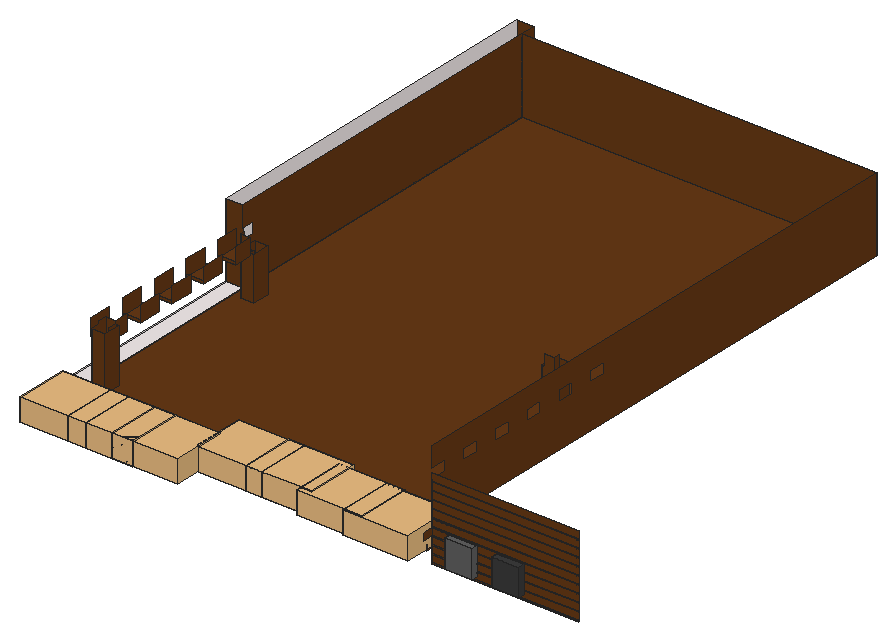
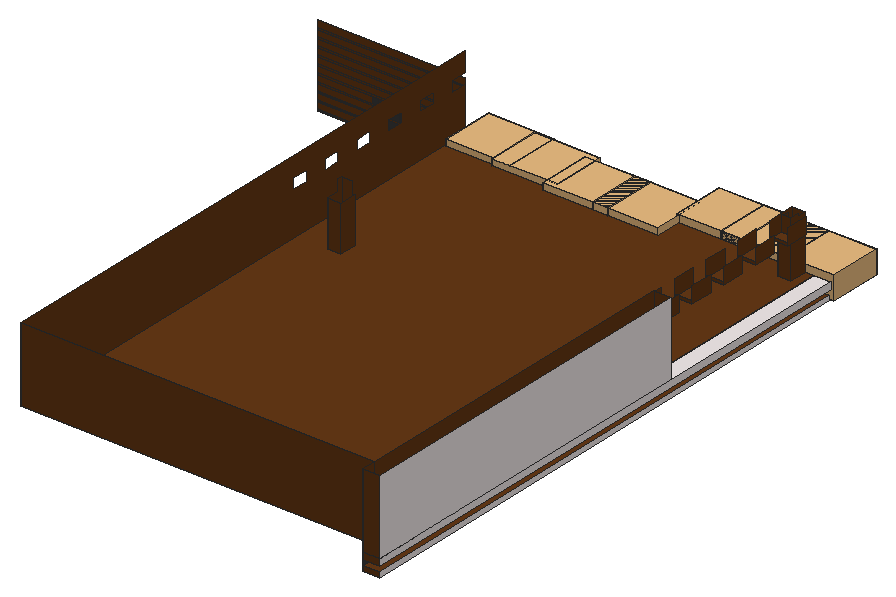
# SketchUp Ruby script. Lengths in inches.
U = 1.inch
M = Sketchup.active_model
def pt(a) = Geom::Point3d.new(a.map { |v| v * U })
def face(e, loops, mat)
  f = e.add_face(loops[0].map { |a| pt(a) })
  loops[1..].each { |l| e.add_face(l.map { |a| pt(a) }).erase! }
  f.material = f.back_material = mat if mat
  f
end
# faces: each face lists its corners as indices into pts; further lists are holes
def faces(e, pts, list, mat = nil) = list.each { |f| face(e, (f[0].is_a?(Array) ? f : [f]).map { |l| l.map { |i| pts[i] } }, mat) }
# xy, xz, yz: faces in a plane at the given z, y or x. An outline is a flat list of corners, or four numbers for a rectangle; further outlines are holes
def ring(l) = l.size == 4 ? [[l[0], l[1]], [l[2], l[1]], [l[2], l[3]], [l[0], l[3]]] : l.each_slice(2).to_a
def flat(e, list, mat, &to3) = list.each { |f| face(e, (f[0].is_a?(Array) ? f : [f]).map { |l| ring(l).map { |u, v| to3.(u, v) } }, mat) }
def xy(e, z, list, mat = nil) = flat(e, list, mat) { |x, y| [x, y, z] }
def xz(e, y, list, mat = nil) = flat(e, list, mat) { |x, z| [x, y, z] }
def yz(e, x, list, mat = nil) = flat(e, list, mat) { |y, z| [x, y, z] }
def lines(e, pts, list) = list.each { |a, b| e.add_line(pt(pts[a]), pt(pts[b])) }
# prism: a flat outline (further loops are holes) pulled along v
def prism(e, loops, v, mat = nil)
  f = face(e, loops, mat); d = Geom::Vector3d.new(v.map { |x| x * U })
  f.pushpull(f.normal.samedirection?(d) ? d.length : -d.length)
end
def box(e, o, s, mat = nil) = prism(e, [[o, [o[0] + s[0], o[1], o[2]], [o[0] + s[0], o[1] + s[1], o[2]], [o[0], o[1] + s[1], o[2]]]], [0, 0, s[2]], mat)
def at(x, y, z, deg = 0) = Geom::Transformation.translation(pt([x, y, z])) * Geom::Transformation.rotation(ORIGIN, Z_AXIS, deg.degrees)
def axes(o, x, y, z) = Geom::Transformation.new([*x, 0, *y, 0, *z, 0, *pt(o).to_a, 1])
def part(name) = M.definitions.add(name)
# library, detail: a bought-in or finely detailed component or shape, given as its bounding box
def library(name, o, s) = part(name).tap { |d| box(d.entities, o, s) }
def detail(e, o, s) = box(e.add_group.entities, o, s)
def put(e, d, t, mat = nil) = e.add_instance(d, t).tap { |i| i.material = mat if mat }
def group(e, t, mat = nil) = e.add_group.tap { |g| g.transformation = t; g.material = mat if mat }.entities
root = M.entities
M.materials.add("Generic").color = [102, 57, 22]
M.materials.add("Generic\#1").color = [96, 96, 96]
M.materials.add("Generic\#2").color = [59, 59, 59]
M.materials.add("Generic\#3").color = [243, 235, 235]
c1 = library("Plante \#58",[-0.43,-1.58,0],[20.84,18.06,17.59])
xy(root,434.875,[[288.56,54.375,403,54.68]],"Generic")
xy(root,435.875,[[288.56,54.375,403,54.68]],"Generic")
xy(root,438.4375,[[302.57,49.5625,323.88,54.375]],"Generic\#1")
xy(root,438.4375,[[339.38,49.5625,360.7,54.375]],"Generic\#2")
xy(root,441.1875,[[288.56,54.375,302.57,54.68],[323.88,54.375,339.38,54.68],[360.7,54.375,403,54.68]],"Generic")
xy(root,442.1875,[[288.56,54.375,302.57,54.68],[323.88,54.375,339.38,54.68],[360.7,54.375,403,54.68]],"Generic")
xy(root,442.58,[[200.32,54.375,201.05,62.9375],[217.69,54.375,218.42,62.9375],[248.26,54.375,248.99,62.9375],[265.63,54.375,266.36,62.9375]],"Generic")
xy(root,443.48,[[200.27,54.375,201.1,58.5625],[217.64,54.375,218.48,58.5625],[248.2,54.375,249.04,58.5625],[265.58,54.375,266.41,58.5625]],"Generic")
xy(root,446.16,[[1.33,49.51,0,498.375,13.1875,498.375,13.1875,54.375,288.56,54.375,288.56,49.625,60.27,49.625,48.53,49.51],[13.1875,54.375,288.56,58.5625]],"Generic")
xy(root,447.5,[[288.56,54.375,302.57,54.68],[323.88,54.375,339.38,54.68],[360.7,54.375,403,54.68]],"Generic")
xy(root,448.5,[[288.56,54.375,302.57,54.68],[323.88,54.375,339.38,54.68],[360.7,54.375,403,54.68]],"Generic")
xy(root,449.97,[[1.33,49.51,48.53,49.51,60.27,49.625,288.56,49.625,288.56,54.375,13.1875,54.375,13.1875,498.375,0,498.375]],"Generic")
xy(root,451.375,[[47.2,40.9375,60.27,47.4375]])
xy(root,453.8125,[[288.56,54.375,302.57,54.68],[323.88,54.375,339.38,54.68],[360.7,54.375,403,54.68]],"Generic")
xy(root,454.8125,[[288.56,54.375,302.57,54.68],[323.88,54.375,339.38,54.68],[360.7,54.375,403,54.68]],"Generic")
xy(root,459.5,[[[13.1875,54.375,288.56,486.875],[19.57,60.38,30.01,73.95],[19.57,205.01,30.01,218.57],[253.89,205.01,264.32,218.57]],[0,215.5,13.1875,498.375]],"Generic")
xy(root,459.75,[[302.57,49.5625,323.88,54.375]],"Generic\#1")
xy(root,459.75,[[339.38,49.5625,360.7,54.375]],"Generic\#2")
xy(root,460.125,[[288.56,54.375,403,54.68]],"Generic")
xy(root,461.125,[[288.56,54.375,403,54.68]],"Generic")
xy(root,466.4375,[[288.56,54.375,403,54.68]],"Generic")
xy(root,467.4375,[[288.56,54.375,403,54.68]],"Generic")
xy(root,472.75,[[288.56,54.375,403,54.68]],"Generic")
xy(root,473.75,[[288.56,54.375,403,54.68]],"Generic")
xy(root,479.0625,[[288.56,54.375,403,54.68]],"Generic")
xy(root,480.0625,[[288.56,54.375,403,54.68]],"Generic")
xy(root,485.375,[[288.56,54.375,403,54.68]],"Generic")
xy(root,486.375,[[288.56,54.375,403,54.68]],"Generic")
xy(root,491.3125,[[13.1875,67.5625,27.12,85.25],[13.1875,98.4375,27.12,116.125],[13.1875,129.3125,27.12,147],[13.1875,160.1875,27.12,177.875],[13.1875,191.0625,27.12,208.75]],"Generic")
xy(root,491.6875,[[288.56,54.375,403,54.68]],"Generic")
xy(root,492.6875,[[288.56,54.375,403,54.68]],"Generic")
xz(root,47.4375,[[47.2,451.375,60.27,454],[47.2,454,60.27,459.5]])
xz(root,49.51,[[1.33,446.16,48.53,449.97]],"Generic\#3")
xz(root,49.5625,[[302.57,438.4375,323.88,459.75]],"Generic\#1")
xz(root,49.5625,[[339.38,438.4375,360.7,459.75]],"Generic\#2")
xz(root,49.625,[[60.27,446.16,288.56,449.97]],"Generic\#3")
xz(root,54.375,[[288.56,435.875,403,435.875,403,441.1875,360.7,441.1875,360.7,438.4375,339.38,438.4375,339.38,441.1875,323.88,441.1875,323.88,438.4375,302.57,438.4375,302.57,441.1875,288.56,441.1875],[302.57,441.1875,323.88,442.1875],[339.38,441.1875,360.7,442.1875],[288.56,442.1875,302.57,447.5],[323.88,442.1875,339.38,447.5],
  [360.7,442.1875,403,447.5],[13.1875,446.16,288.56,449.97],[302.57,447.5,323.88,448.5],[339.38,447.5,360.7,448.5],[288.56,448.5,302.57,453.8125],
  [323.88,448.5,339.38,453.8125],[360.7,448.5,403,453.8125],[302.57,453.8125,323.88,454.8125],[339.38,453.8125,360.7,454.8125],[13.1875,454,288.56,459.5],
  [288.56,454.8125,302.57,454.8125,302.57,459.75,323.88,459.75,323.88,454.8125,339.38,454.8125,339.38,459.75,360.7,459.75,360.7,454.8125,403,454.8125,403,460.125,288.56,460.125],[288.56,461.125,403,466.4375],[288.56,467.4375,403,472.75],[288.56,473.75,403,479.0625],[288.56,480.0625,403,485.375],
  [288.56,486.375,403,491.6875],[288.56,492.6875,403,498]],"Generic")
xz(root,54.375,[[13.1875,449.97,288.56,454]],"Generic\#2")
xz(root,54.68,[[288.56,434.875,403,435.875],[288.56,441.1875,302.57,442.1875],[323.88,441.1875,339.38,442.1875],[360.7,441.1875,403,442.1875],[288.56,447.5,302.57,448.5],
  [323.88,447.5,339.38,448.5],[360.7,447.5,403,448.5],[288.56,453.8125,302.57,454.8125],[323.88,453.8125,339.38,454.8125],[360.7,453.8125,403,454.8125],
  [288.56,460.125,403,461.125],[288.56,466.4375,403,467.4375],[288.56,472.75,403,473.75],[288.56,479.0625,403,480.0625],[288.56,485.375,403,486.375],
  [288.56,491.6875,403,492.6875]],"Generic")
xz(root,60.38,[[19.57,459.5,30.01,501.48]],"Generic")
xz(root,67.5625,[[13.1875,491.3125,27.12,493.4375]],"Generic")
xz(root,73.95,[[19.57,459.5,19.57,503.72,27.12,503.72,27.12,501.48,30.01,501.48,30.01,459.5]],"Generic")
xz(root,85.25,[[13.1875,491.3125,27.12,493.4375]],"Generic")
xz(root,98.4375,[[13.1875,491.3125,27.12,493.4375]],"Generic")
xz(root,116.125,[[13.1875,491.3125,27.12,493.4375]],"Generic")
xz(root,129.3125,[[13.1875,491.3125,27.12,493.4375]],"Generic")
xz(root,147,[[13.1875,491.3125,27.12,493.4375]],"Generic")
xz(root,160.1875,[[13.1875,491.3125,27.12,493.4375]],"Generic")
xz(root,177.875,[[13.1875,491.3125,27.12,493.4375]],"Generic")
xz(root,191.0625,[[13.1875,491.3125,27.12,493.4375]],"Generic")
xz(root,205.01,[[19.57,459.5,30.01,459.5,30.01,493.22,27.12,493.22,27.12,503.72,19.57,503.72],[253.89,459.5,264.32,459.5,264.32,503.72,256.5625,503.72,256.5625,494.78,253.89,494.78]],"Generic")
xz(root,208.75,[[13.1875,491.3125,13.1875,493.4375,19.57,493.4375,19.57,493.22,27.12,493.22,27.12,491.3125]],"Generic")
xz(root,215.5,[[0,459.5,13.1875,517.125]],"Generic")
xz(root,218.57,[[19.57,459.5,30.01,493.22],[253.89,459.5,264.32,494.78]],"Generic")
xz(root,486.875,[[13.1875,459.5,288.56,517.125]],"Generic")
xz(root,498.375,[[0,446.16,13.1875,449.97],[0,454,13.1875,459.5],[0,459.5,13.1875,517.125]],"Generic")
yz(root,0,[[215.5,459.5,498.375,517.125]],"Generic\#3")
yz(root,13.1875,[[54.375,446.16,498.375,449.97],[54.375,454,486.875,459.5],[486.875,454,498.375,459.5],[215.5,459.5,486.875,459.5,486.875,517.125,215.5,517.125,215.5,501.6,224.75,501.6,224.75,493.4375,215.5,493.4375],[486.875,459.5,498.375,517.125],
  [67.5625,491.3125,85.25,503.72],[98.4375,491.3125,116.125,503.72],[129.3125,491.3125,147,503.72],[160.1875,491.3125,177.875,503.72],[191.0625,491.3125,208.75,503.72]],"Generic")
yz(root,13.1875,[[54.375,449.97,498.375,454]],"Generic\#2")
yz(root,19.57,[[60.38,459.5,60.38,501.48,67.5625,501.48,67.5625,503.72,73.95,503.72,73.95,459.5],[205.01,459.5,205.01,503.72,208.75,503.72,208.75,493.22,218.57,493.22,218.57,459.5]],"Generic")
yz(root,27.12,[[67.5625,491.3125,85.25,491.3125,85.25,503.72,73.95,503.72,73.95,501.48,67.5625,501.48],[98.4375,491.3125,116.125,503.72],[129.3125,491.3125,147,503.72],[160.1875,491.3125,177.875,503.72],[191.0625,491.3125,208.75,491.3125,208.75,493.22,205.01,493.22,205.01,503.72,191.0625,503.72]],"Generic")
yz(root,30.01,[[60.38,459.5,73.95,501.48],[205.01,459.5,218.57,493.22]],"Generic")
yz(root,253.89,[[205.01,459.5,218.57,494.78]],"Generic")
yz(root,264.32,[[205.01,459.5,218.57,459.5,218.57,494.78,208.75,494.78,208.75,503.72,205.01,503.72]],"Generic")
yz(root,288.56,[[54.375,434.875,54.68,435.875],[54.68,434.875,58.5625,435.875],[54.375,435.875,58.5625,441.1875],[54.375,441.1875,54.68,442.1875],[54.68,441.1875,58.5625,442.1875],
  [54.375,442.1875,58.5625,446.16],[54.375,447.5,54.68,448.5],[54.375,453.8125,54.68,454.8125],[47.4375,454,54.375,459.5],[[54.375,459.5,54.375,460.125,54.68,460.125,54.68,461.125,54.375,461.125,54.375,466.4375,54.68,466.4375,54.68,467.4375,54.375,467.4375,54.375,472.75,54.68,472.75,54.68,473.75,54.375,473.75,54.375,479.0625,54.68,479.0625,54.68,480.0625,54.375,480.0625,54.375,485.375,54.68,485.375,54.68,486.375,54.375,486.375,54.375,491.6875,54.68,491.6875,54.68,492.6875,54.375,492.6875,54.375,493.4375,67.5625,493.4375,67.5625,501.6,54.375,501.6,54.375,504.3125,54.68,504.3125,54.68,505.3125,54.375,505.3125,54.375,510.625,54.68,510.625,54.68,511.625,54.375,511.625,54.375,517.125,486.875,517.125,486.875,459.5],[208.75,493.4375,221.9375,501.6],[177.875,493.4375,191.0625,501.6],[147,493.4375,160.1875,501.6],[116.125,493.4375,129.3125,501.6],[85.25,493.4375,98.4375,501.6]]],"Generic")
yz(root,302.57,[[54.375,441.1875,54.68,442.1875],[54.375,447.5,54.68,448.5],[54.375,453.8125,54.68,454.8125]],"Generic")
yz(root,302.57,[[49.5625,438.4375,54.375,459.75]],"Generic\#1")
yz(root,323.88,[[54.375,441.1875,54.68,442.1875],[54.375,447.5,54.68,448.5],[54.375,453.8125,54.68,454.8125]],"Generic")
yz(root,323.88,[[49.5625,438.4375,54.375,459.75]],"Generic\#1")
yz(root,339.38,[[54.375,441.1875,54.68,442.1875],[54.375,447.5,54.68,448.5],[54.375,453.8125,54.68,454.8125]],"Generic")
yz(root,339.38,[[49.5625,438.4375,54.375,459.75]],"Generic\#2")
yz(root,360.7,[[54.375,441.1875,54.68,442.1875],[54.375,447.5,54.68,448.5],[54.375,453.8125,54.68,454.8125]],"Generic")
yz(root,360.7,[[49.5625,438.4375,54.375,459.75]],"Generic\#2")
yz(root,403,[[54.375,434.875,54.68,435.875],[54.375,441.1875,54.68,442.1875],[54.375,447.5,54.68,448.5],[54.375,453.8125,54.68,454.8125],[54.375,460.125,54.68,461.125],
  [54.375,466.4375,54.68,467.4375],[54.375,472.75,54.68,473.75],[54.375,479.0625,54.68,480.0625],[54.375,485.375,54.68,486.375],[54.375,491.6875,54.68,492.6875]],"Generic")
p = [[195.44,54.375,432.86],[195.87,54.375,432.27],[195.87,62.9375,432.27],[195.44,62.9375,432.86],[205.5,54.375,432.27],[205.93,54.375,432.86],
  [205.93,62.9375,432.86],[205.5,62.9375,432.27],[212.81,54.375,432.86],[213.25,54.375,432.27],[213.25,62.9375,432.27],[212.81,62.9375,432.86],
  [222.87,54.375,432.27],[223.31,54.375,432.86],[223.31,62.9375,432.86],[222.87,62.9375,432.27],[243.37,54.375,432.86],[243.81,54.375,432.27],
  [243.81,62.9375,432.27],[243.37,62.9375,432.86],[253.43,54.375,432.27],[253.87,54.375,432.86],[253.87,62.9375,432.86],[253.43,62.9375,432.27],
  [260.75,54.375,432.86],[261.18,54.375,432.27],[261.18,62.9375,432.27],[260.75,62.9375,432.86],[270.81,54.375,432.27],[271.25,54.375,432.86],
  [271.25,62.9375,432.86],[270.81,62.9375,432.27],[194.26,54.375,433.08],[194.68,54.375,432.36],[194.68,58.5625,432.36],[194.26,58.5625,433.08],
  [206.6875,54.375,432.36],[207.11,54.375,433.08],[207.11,58.5625,433.08],[206.6875,58.5625,432.36],[211.64,54.375,433.08],[212.05,54.375,432.36],
  [212.05,58.5625,432.36],[211.64,58.5625,433.08],[224.0625,54.375,432.36],[224.48,54.375,433.08],[224.48,58.5625,433.08],[224.0625,58.5625,432.36],
  [242.2,54.375,433.08],[242.62,54.375,432.36],[242.62,58.5625,432.36],[242.2,58.5625,433.08],[254.625,54.375,432.36],[255.04,54.375,433.08],
  [255.04,58.5625,433.08],[254.625,58.5625,432.36],[259.57,54.375,433.08],[259.99,54.375,432.36],[259.99,58.5625,432.36],[259.57,58.5625,433.08],
  [272,54.375,432.36],[272.42,54.375,433.08],[272.42,58.5625,433.08],[272,58.5625,432.36],[195.07,54.375,433.49],[195.07,62.9375,433.49],
  [206.3,54.375,433.49],[206.3,62.9375,433.49],[212.44,54.375,433.49],[212.44,62.9375,433.49],[223.67,54.375,433.49],[223.67,62.9375,433.49],
  [243.01,54.375,433.49],[243.01,62.9375,433.49],[254.24,54.375,433.49],[254.24,62.9375,433.49],[260.38,54.375,433.49],[260.38,62.9375,433.49],
  [271.61,54.375,433.49],[271.61,62.9375,433.49],[193.93,54.375,433.85],[193.93,58.5625,433.85],[207.4375,54.375,433.85],[207.4375,58.5625,433.85],
  [211.31,54.375,433.85],[211.31,58.5625,433.85],[224.8125,54.375,433.85],[224.8125,58.5625,433.85],[241.87,54.375,433.85],[241.87,58.5625,433.85],
  [255.375,54.375,433.85],[255.375,58.5625,433.85],[259.24,54.375,433.85],[259.24,58.5625,433.85],[272.75,54.375,433.85],[272.75,58.5625,433.85],
  [194.78,54.375,434.16],[194.78,62.9375,434.16],[206.59,54.375,434.16],[206.59,62.9375,434.16],[212.16,54.375,434.16],[212.16,62.9375,434.16],
  [223.96,54.375,434.16],[223.96,62.9375,434.16],[242.72,54.375,434.16],[242.72,62.9375,434.16],[254.53,54.375,434.16],[254.53,62.9375,434.16],
  [260.09,54.375,434.16],[260.09,62.9375,434.16],[271.9,54.375,434.16],[271.9,62.9375,434.16],[193.69,54.375,434.65],[193.69,58.5625,434.65],
  [207.68,54.375,434.65],[207.68,58.5625,434.65],[211.07,54.375,434.65],[211.07,58.5625,434.65],[225.05,54.375,434.65],[225.05,58.5625,434.65],
  [241.63,54.375,434.65],[241.63,58.5625,434.65],[255.62,54.375,434.65],[255.62,58.5625,434.65],[259,54.375,434.65],[259,58.5625,434.65],
  [272.99,54.375,434.65],[272.99,58.5625,434.65],[194.57,54.375,434.86],[194.57,62.9375,434.86],[206.8,54.375,434.86],[206.8,62.9375,434.86],
  [211.95,54.375,434.86],[211.95,62.9375,434.86],[224.17,54.375,434.86],[224.17,62.9375,434.86],[242.51,54.375,434.86],[242.51,62.9375,434.86],
  [254.73,54.375,434.86],[254.73,62.9375,434.86],[259.88,54.375,434.86],[259.88,62.9375,434.86],[272.11,54.375,434.86],[272.11,62.9375,434.86],
  [193.55,54.375,435.47],[193.55,58.5625,435.47],[207.82,54.375,435.47],[207.82,58.5625,435.47],[210.92,54.375,435.47],[210.92,58.5625,435.47],
  [225.2,54.375,435.47],[225.2,58.5625,435.47],[241.48,54.375,435.47],[241.48,58.5625,435.47],[255.76,54.375,435.47],[255.76,58.5625,435.47],
  [258.86,54.375,435.47],[258.86,58.5625,435.47],[273.14,54.375,435.47],[273.14,58.5625,435.47],[194.44,54.375,435.58],[194.44,62.9375,435.58],
  [206.92,54.375,435.58],[206.92,62.9375,435.58],[211.82,54.375,435.58],[211.82,62.9375,435.58],[224.3,54.375,435.58],[224.3,62.9375,435.58],
  [242.38,54.375,435.58],[242.38,62.9375,435.58],[254.86,54.375,435.58],[254.86,62.9375,435.58],[259.76,54.375,435.58],[259.76,62.9375,435.58],
  [272.24,54.375,435.58],[272.24,62.9375,435.58],[193.5,54.375,436.31],[193.5,58.5625,436.31],[207.87,54.375,436.31],[207.87,58.5625,436.31],
  [210.87,54.375,436.31],[210.87,58.5625,436.31],[225.25,54.375,436.31],[225.25,58.5625,436.31],[241.43,54.375,436.31],[241.43,58.5625,436.31],
  [255.81,54.375,436.31],[255.81,58.5625,436.31],[258.81,54.375,436.31],[258.81,58.5625,436.31],[273.18,54.375,436.31],[273.18,58.5625,436.31],
  [194.4,54.375,436.31],[194.4,62.9375,436.31],[206.97,54.375,436.31],[206.97,62.9375,436.31],[211.78,54.375,436.31],[211.78,62.9375,436.31],
  [224.34,54.375,436.31],[224.34,62.9375,436.31],[242.34,54.375,436.31],[242.34,62.9375,436.31],[254.9,54.375,436.31],[254.9,62.9375,436.31],
  [259.71,54.375,436.31],[259.71,62.9375,436.31],[272.28,54.375,436.31],[272.28,62.9375,436.31],[193.55,54.375,437.14],[193.55,58.5625,437.14],
  [194.44,54.375,437.04],[194.44,62.9375,437.04],[206.92,54.375,437.04],[206.92,62.9375,437.04],[207.82,54.375,437.14],[207.82,58.5625,437.14],
  [210.92,54.375,437.14],[210.92,58.5625,437.14],[211.82,54.375,437.04],[211.82,62.9375,437.04],[224.3,54.375,437.04],[224.3,62.9375,437.04],
  [225.2,54.375,437.14],[225.2,58.5625,437.14],[241.48,54.375,437.14],[241.48,58.5625,437.14],[242.38,54.375,437.04],[242.38,62.9375,437.04],
  [254.86,54.375,437.04],[254.86,62.9375,437.04],[255.76,54.375,437.14],[255.76,58.5625,437.14],[258.86,54.375,437.14],[258.86,58.5625,437.14],
  [259.76,54.375,437.04],[259.76,62.9375,437.04],[272.24,54.375,437.04],[272.24,62.9375,437.04],[273.14,54.375,437.14],[273.14,58.5625,437.14],
  [194.57,54.375,437.76],[194.57,62.9375,437.76],[206.8,54.375,437.76],[206.8,62.9375,437.76],[211.95,54.375,437.76],[211.95,62.9375,437.76],
  [224.17,54.375,437.76],[224.17,62.9375,437.76],[242.51,54.375,437.76],[242.51,62.9375,437.76],[254.73,54.375,437.76],[254.73,62.9375,437.76],
  [259.88,54.375,437.76],[259.88,62.9375,437.76],[272.11,54.375,437.76],[272.11,62.9375,437.76],[193.69,54.375,437.97],[193.69,58.5625,437.97],
  [207.68,54.375,437.97],[207.68,58.5625,437.97],[211.07,54.375,437.97],[211.07,58.5625,437.97],[225.05,54.375,437.97],[225.05,58.5625,437.97],
  [241.63,54.375,437.97],[241.63,58.5625,437.97],[255.62,54.375,437.97],[255.62,58.5625,437.97],[259,54.375,437.97],[259,58.5625,437.97],
  [272.99,54.375,437.97],[272.99,58.5625,437.97],[194.78,54.375,438.46],[194.78,62.9375,438.46],[206.59,54.375,438.46],[206.59,62.9375,438.46],
  [212.16,54.375,438.46],[212.16,62.9375,438.46],[223.96,54.375,438.46],[223.96,62.9375,438.46],[242.72,54.375,438.46],[242.72,62.9375,438.46],
  [254.53,54.375,438.46],[254.53,62.9375,438.46],[260.09,54.375,438.46],[260.09,62.9375,438.46],[271.9,54.375,438.46],[271.9,62.9375,438.46],
  [193.93,54.375,438.77],[193.93,58.5625,438.77],[207.4375,54.375,438.77],[207.4375,58.5625,438.77],[211.31,54.375,438.77],[211.31,58.5625,438.77],
  [224.8125,54.375,438.77],[224.8125,58.5625,438.77],[241.87,54.375,438.77],[241.87,58.5625,438.77],[255.375,54.375,438.77],[255.375,58.5625,438.77],
  [259.24,54.375,438.77],[259.24,58.5625,438.77],[272.75,54.375,438.77],[272.75,58.5625,438.77],[195.07,54.375,439.13],[195.07,62.9375,439.13],
  [206.3,54.375,439.13],[206.3,62.9375,439.13],[212.44,54.375,439.13],[212.44,62.9375,439.13],[223.67,54.375,439.13],[223.67,62.9375,439.13],
  [243.01,54.375,439.13],[243.01,62.9375,439.13],[254.24,54.375,439.13],[254.24,62.9375,439.13],[260.38,54.375,439.13],[260.38,62.9375,439.13],
  [271.61,54.375,439.13],[271.61,62.9375,439.13],[194.26,54.375,439.53],[194.26,58.5625,439.53],[207.11,54.375,439.53],[207.11,58.5625,439.53],
  [211.64,54.375,439.53],[211.64,58.5625,439.53],[224.48,54.375,439.53],[224.48,58.5625,439.53],[242.2,54.375,439.53],[242.2,58.5625,439.53],
  [255.04,54.375,439.53],[255.04,58.5625,439.53],[259.57,54.375,439.53],[259.57,58.5625,439.53],[272.42,54.375,439.53],[272.42,58.5625,439.53],
  [195.44,54.375,439.76],[195.44,62.9375,439.76],[205.93,54.375,439.76],[205.93,62.9375,439.76],[212.81,54.375,439.76],[212.81,62.9375,439.76],
  [223.31,54.375,439.76],[223.31,62.9375,439.76],[243.37,54.375,439.76],[243.37,62.9375,439.76],[253.87,54.375,439.76],[253.87,62.9375,439.76],
  [260.75,54.375,439.76],[260.75,62.9375,439.76],[271.25,54.375,439.76],[271.25,62.9375,439.76],[194.68,54.375,440.26],[194.68,58.5625,440.26],
  [206.6875,54.375,440.26],[206.6875,58.5625,440.26],[212.05,54.375,440.26],[212.05,58.5625,440.26],[224.0625,54.375,440.26],[224.0625,58.5625,440.26],
  [242.62,54.375,440.26],[242.62,58.5625,440.26],[254.625,54.375,440.26],[254.625,58.5625,440.26],[259.99,54.375,440.26],[259.99,58.5625,440.26],
  [272,54.375,440.26],[272,58.5625,440.26],[195.87,54.375,440.35],[195.87,62.9375,440.35],[205.5,54.375,440.35],[205.5,62.9375,440.35],
  [213.25,54.375,440.35],[213.25,62.9375,440.35],[222.87,54.375,440.35],[222.87,62.9375,440.35],[243.81,54.375,440.35],[243.81,62.9375,440.35],
  [253.43,54.375,440.35],[253.43,62.9375,440.35],[261.18,54.375,440.35],[261.18,62.9375,440.35],[270.81,54.375,440.35],[270.81,62.9375,440.35],
  [195.18,54.375,440.93],[195.18,58.5625,440.93],[196.37,54.375,440.88],[196.37,62.9375,440.88],[205,54.375,440.88],[205,62.9375,440.88],
  [206.19,54.375,440.93],[206.19,58.5625,440.93],[212.55,54.375,440.93],[212.55,58.5625,440.93],[213.75,54.375,440.88],[213.75,62.9375,440.88],
  [222.37,54.375,440.88],[222.37,62.9375,440.88],[223.57,54.375,440.93],[223.57,58.5625,440.93],[243.12,54.375,440.93],[243.12,58.5625,440.93],
  [244.31,54.375,440.88],[244.31,62.9375,440.88],[252.93,54.375,440.88],[252.93,62.9375,440.88],[254.13,54.375,440.93],[254.13,58.5625,440.93],
  [260.49,54.375,440.93],[260.49,58.5625,440.93],[261.69,54.375,440.88],[261.69,62.9375,440.88],[270.31,54.375,440.88],[270.31,62.9375,440.88],
  [271.5,54.375,440.93],[271.5,58.5625,440.93],[195.75,54.375,441.54],[195.75,58.5625,441.54],[196.93,54.375,441.35],[196.93,62.9375,441.35],
  [204.4375,54.375,441.35],[204.4375,62.9375,441.35],[205.62,54.375,441.54],[205.62,58.5625,441.54],[213.125,54.375,441.54],[213.125,58.5625,441.54],
  [214.31,54.375,441.35],[214.31,62.9375,441.35],[221.8125,54.375,441.35],[221.8125,62.9375,441.35],[222.99,54.375,441.54],[222.99,58.5625,441.54],
  [243.6875,54.375,441.54],[243.6875,58.5625,441.54],[244.87,54.375,441.35],[244.87,62.9375,441.35],[252.375,54.375,441.35],[252.375,62.9375,441.35],
  [253.55,54.375,441.54],[253.55,58.5625,441.54],[261.0625,54.375,441.54],[261.0625,58.5625,441.54],[262.25,54.375,441.35],[262.25,62.9375,441.35],
  [269.75,54.375,441.35],[269.75,62.9375,441.35],[270.93,54.375,441.54],[270.93,58.5625,441.54],[197.54,54.375,441.75],[197.54,62.9375,441.75],
  [203.83,54.375,441.75],[203.83,62.9375,441.75],[214.92,54.375,441.75],[214.92,62.9375,441.75],[221.2,54.375,441.75],[221.2,62.9375,441.75],
  [245.48,54.375,441.75],[245.48,62.9375,441.75],[251.76,54.375,441.75],[251.76,62.9375,441.75],[262.86,54.375,441.75],[262.86,62.9375,441.75],
  [269.14,54.375,441.75],[269.14,62.9375,441.75],[196.39,54.375,442.07],[196.39,58.5625,442.07],[204.98,54.375,442.07],[204.98,58.5625,442.07],
  [213.77,54.375,442.07],[213.77,58.5625,442.07],[222.35,54.375,442.07],[222.35,58.5625,442.07],[244.33,54.375,442.07],[244.33,58.5625,442.07],
  [252.91,54.375,442.07],[252.91,58.5625,442.07],[261.7,54.375,442.07],[261.7,58.5625,442.07],[270.29,54.375,442.07],[270.29,58.5625,442.07],
  [198.2,54.375,442.08],[198.2,62.9375,442.08],[203.17,54.375,442.08],[203.17,62.9375,442.08],[215.57,54.375,442.08],[215.57,62.9375,442.08],
  [220.55,54.375,442.08],[220.55,62.9375,442.08],[246.13,54.375,442.08],[246.13,62.9375,442.08],[251.11,54.375,442.08],[251.11,62.9375,442.08],
  [263.51,54.375,442.08],[263.51,62.9375,442.08],[268.48,54.375,442.08],[268.48,62.9375,442.08],[197.09,54.375,442.53],[197.09,58.5625,442.53],
  [198.88,54.375,442.33],[198.88,62.9375,442.33],[202.49,54.375,442.33],[202.49,62.9375,442.33],[204.28,54.375,442.53],[204.28,58.5625,442.53],
  [214.47,54.375,442.53],[214.47,58.5625,442.53],[216.26,54.375,442.33],[216.26,62.9375,442.33],[219.86,54.375,442.33],[219.86,62.9375,442.33],
  [221.65,54.375,442.53],[221.65,58.5625,442.53],[245.03,54.375,442.53],[245.03,58.5625,442.53],[246.82,54.375,442.33],[246.82,62.9375,442.33],
  [250.42,54.375,442.33],[250.42,62.9375,442.33],[252.22,54.375,442.53],[252.22,58.5625,442.53],[262.4,54.375,442.53],[262.4,58.5625,442.53],
  [264.19,54.375,442.33],[264.19,62.9375,442.33],[267.8,54.375,442.33],[267.8,62.9375,442.33],[269.59,54.375,442.53],[269.59,58.5625,442.53],
  [199.59,54.375,442.5],[199.59,62.9375,442.5],[201.78,54.375,442.5],[201.78,62.9375,442.5],[216.97,54.375,442.5],[216.97,62.9375,442.5],
  [219.15,54.375,442.5],[219.15,62.9375,442.5],[247.53,54.375,442.5],[247.53,62.9375,442.5],[249.71,54.375,442.5],[249.71,62.9375,442.5],
  [264.91,54.375,442.5],[264.91,62.9375,442.5],[267.09,54.375,442.5],[267.09,62.9375,442.5],[197.84,54.375,442.91],[197.84,58.5625,442.91],
  [200.32,54.375,442.58],[200.32,62.9375,442.58],[201.05,54.375,442.58],[201.05,62.9375,442.58],[203.53,54.375,442.91],[203.53,58.5625,442.91],
  [215.21,54.375,442.91],[215.21,58.5625,442.91],[217.69,54.375,442.58],[217.69,62.9375,442.58],[218.42,54.375,442.58],[218.42,62.9375,442.58],
  [220.91,54.375,442.91],[220.91,58.5625,442.91],[245.77,54.375,442.91],[245.77,58.5625,442.91],[248.26,54.375,442.58],[248.26,62.9375,442.58],
  [248.99,54.375,442.58],[248.99,62.9375,442.58],[251.47,54.375,442.91],[251.47,58.5625,442.91],[263.15,54.375,442.91],[263.15,58.5625,442.91],
  [265.63,54.375,442.58],[265.63,62.9375,442.58],[266.36,54.375,442.58],[266.36,62.9375,442.58],[268.84,54.375,442.91],[268.84,58.5625,442.91],
  [198.62,54.375,443.19],[198.62,58.5625,443.19],[202.75,54.375,443.19],[202.75,58.5625,443.19],[216,54.375,443.19],[216,58.5625,443.19],
  [220.12,54.375,443.19],[220.12,58.5625,443.19],[246.56,54.375,443.19],[246.56,58.5625,443.19],[250.68,54.375,443.19],[250.68,58.5625,443.19],
  [263.94,54.375,443.19],[263.94,58.5625,443.19],[268.06,54.375,443.19],[268.06,58.5625,443.19],[199.4375,54.375,443.39],[199.4375,58.5625,443.39],
  [201.93,54.375,443.39],[201.93,58.5625,443.39],[216.8125,54.375,443.39],[216.8125,58.5625,443.39],[219.31,54.375,443.39],[219.31,58.5625,443.39],
  [247.375,54.375,443.39],[247.375,58.5625,443.39],[249.87,54.375,443.39],[249.87,58.5625,443.39],[264.75,54.375,443.39],[264.75,58.5625,443.39],
  [267.24,54.375,443.39],[267.24,58.5625,443.39],[200.27,54.375,443.48],[200.27,58.5625,443.48],[201.1,54.375,443.48],[201.1,58.5625,443.48],
  [217.64,54.375,443.48],[217.64,58.5625,443.48],[218.48,54.375,443.48],[218.48,58.5625,443.48],[248.2,54.375,443.48],[248.2,58.5625,443.48],
  [249.04,54.375,443.48],[249.04,58.5625,443.48],[265.58,54.375,443.48],[265.58,58.5625,443.48],[266.41,54.375,443.48],[266.41,58.5625,443.48],
  [0,498.375,449.97],[0,498.375,446.16],[1.33,49.51,446.16],[1.33,49.51,449.97],[48.53,49.51,446.16],[60.27,49.625,446.16],
  [60.27,49.625,449.97],[48.53,49.51,449.97]]
faces(root,p,[[0,1,2,3],[4,5,6,7],[8,9,10,11],[12,13,14,15],[16,17,18,19],[20,21,22,23],[24,25,26,27],[28,29,30,31],
  [32,33,34,35],[36,37,38,39],[40,41,42,43],[44,45,46,47],[48,49,50,51],[52,53,54,55],[56,57,58,59],[60,61,62,63],
  [64,0,3,65],[5,66,67,6],[68,8,11,69],[13,70,71,14],[72,16,19,73],[21,74,75,22],[76,24,27,77],[29,78,79,30],
  [80,32,35,81],[37,82,83,38],[84,40,43,85],[45,86,87,46],[88,48,51,89],[53,90,91,54],[92,56,59,93],[61,94,95,62],
  [96,64,65,97],[66,98,99,67],[100,68,69,101],[70,102,103,71],[104,72,73,105],[74,106,107,75],[108,76,77,109],[78,110,111,79],
  [112,80,81,113],[82,114,115,83],[116,84,85,117],[86,118,119,87],[120,88,89,121],[90,122,123,91],[124,92,93,125],[94,126,127,95],
  [128,96,97,129],[98,130,131,99],[132,100,101,133],[102,134,135,103],[136,104,105,137],[106,138,139,107],[140,108,109,141],[110,142,143,111],
  [144,112,113,145],[114,146,147,115],[148,116,117,149],[118,150,151,119],[152,120,121,153],[122,154,155,123],[156,124,125,157],[126,158,159,127],
  [160,128,129,161],[130,162,163,131],[164,132,133,165],[134,166,167,135],[168,136,137,169],[138,170,171,139],[172,140,141,173],[142,174,175,143],
  [176,144,145,177],[146,178,179,147],[180,148,149,181],[150,182,183,151],[184,152,153,185],[154,186,187,155],[188,156,157,189],[158,190,191,159],
  [192,160,161,193],[162,194,195,163],[196,164,165,197],[166,198,199,167],[200,168,169,201],[170,202,203,171],[204,172,173,205],[174,206,207,175],
  [208,176,177,209],[210,192,193,211],[194,212,213,195],[178,214,215,179],[216,180,181,217],[218,196,197,219],[198,220,221,199],[182,222,223,183],
  [224,184,185,225],[226,200,201,227],[202,228,229,203],[186,230,231,187],[232,188,189,233],[234,204,205,235],[206,236,237,207],[190,238,239,191],
  [240,210,211,241],[212,242,243,213],[244,218,219,245],[220,246,247,221],[248,226,227,249],[228,250,251,229],[252,234,235,253],[236,254,255,237],
  [256,208,209,257],[214,258,259,215],[260,216,217,261],[222,262,263,223],[264,224,225,265],[230,266,267,231],[268,232,233,269],[238,270,271,239],
  [272,240,241,273],[242,274,275,243],[276,244,245,277],[246,278,279,247],[280,248,249,281],[250,282,283,251],[284,252,253,285],[254,286,287,255],
  [288,256,257,289],[258,290,291,259],[292,260,261,293],[262,294,295,263],[296,264,265,297],[266,298,299,267],[300,268,269,301],[270,302,303,271],
  [304,272,273,305],[274,306,307,275],[308,276,277,309],[278,310,311,279],[312,280,281,313],[282,314,315,283],[316,284,285,317],[286,318,319,287],
  [320,288,289,321],[290,322,323,291],[324,292,293,325],[294,326,327,295],[328,296,297,329],[298,330,331,299],[332,300,301,333],[302,334,335,303],
  [336,304,305,337],[306,338,339,307],[340,308,309,341],[310,342,343,311],[344,312,313,345],[314,346,347,315],[348,316,317,349],[318,350,351,319],
  [352,320,321,353],[322,354,355,323],[356,324,325,357],[326,358,359,327],[360,328,329,361],[330,362,363,331],[364,332,333,365],[334,366,367,335],
  [368,336,337,369],[338,370,371,339],[372,340,341,373],[342,374,375,343],[376,344,345,377],[346,378,379,347],[380,348,349,381],[350,382,383,351],
  [384,352,353,385],[386,368,369,387],[370,388,389,371],[354,390,391,355],[392,356,357,393],[394,372,373,395],[374,396,397,375],[358,398,399,359],
  [400,360,361,401],[402,376,377,403],[378,404,405,379],[362,406,407,363],[408,364,365,409],[410,380,381,411],[382,412,413,383],[366,414,415,367],
  [416,384,385,417],[418,386,387,419],[388,420,421,389],[390,422,423,391],[424,392,393,425],[426,394,395,427],[396,428,429,397],[398,430,431,399],
  [432,400,401,433],[434,402,403,435],[404,436,437,405],[406,438,439,407],[440,408,409,441],[442,410,411,443],[412,444,445,413],[414,446,447,415],
  [448,418,419,449],[420,450,451,421],[452,426,427,453],[428,454,455,429],[456,434,435,457],[436,458,459,437],[460,442,443,461],[444,462,463,445],
  [464,416,417,465],[422,466,467,423],[468,424,425,469],[430,470,471,431],[472,432,433,473],[438,474,475,439],[476,440,441,477],[446,478,479,447],
  [480,448,449,481],[450,482,483,451],[484,452,453,485],[454,486,487,455],[488,456,457,489],[458,490,491,459],[492,460,461,493],[462,494,495,463],
  [496,464,465,497],[498,480,481,499],[482,500,501,483],[466,502,503,467],[504,468,469,505],[506,484,485,507],[486,508,509,487],[470,510,511,471],
  [512,472,473,513],[514,488,489,515],[490,516,517,491],[474,518,519,475],[520,476,477,521],[522,492,493,523],[494,524,525,495],[478,526,527,479],
  [528,498,499,529],[500,530,531,501],[532,506,507,533],[508,534,535,509],[536,514,515,537],[516,538,539,517],[540,522,523,541],[524,542,543,525],
  [544,496,497,545],[546,528,529,547],[530,548,549,531],[502,550,551,503],[552,504,505,553],[554,532,533,555],[534,556,557,535],[510,558,559,511],
  [560,512,513,561],[562,536,537,563],[538,564,565,539],[518,566,567,519],[568,520,521,569],[570,540,541,571],[542,572,573,543],[526,574,575,527],
  [576,544,545,577],[550,578,579,551],[580,552,553,581],[558,582,583,559],[584,560,561,585],[566,586,587,567],[588,568,569,589],[574,590,591,575],
  [592,576,577,593],[578,594,595,579],[596,580,581,597],[582,598,599,583],[600,584,585,601],[586,602,603,587],[604,588,589,605],[590,606,607,591],
  [608,592,593,609],[594,610,611,595],[612,596,597,613],[598,614,615,599],[616,600,601,617],[602,618,619,603],[620,604,605,621],[606,622,623,607],
  [628,629,630,631]],"Generic")
faces(root,p,[[624,625,626,627]],"Generic\#3")
put(root,c1,axes([238.36,36,446.43],[2.44,0,0],[0,2.3,0],[0,0,1]))
put(root,c1,axes([201.22,37.38,446.625],[2.44,0,0],[0,2.3,0],[0,0,1]))
put(root,c1,axes([158.44,41.77,446.75],[2.44,0,0],[0,2.3,0],[0,0,1]))
put(root,c1,axes([119.57,41.77,446.75],[2.44,0,0],[0,2.3,0],[0,0,1]))
put(root,c1,axes([70.35,21.7,447.23],[2.44,0,0],[0,2.3,0],[0,0,1]))
put(root,c1,axes([35.9,21.7,447.23],[2.44,0,0],[0,2.3,0],[0,0,1]))
put(root,c1,axes([-1.01,21.7,447.23],[2.44,0,0],[0,2.3,0],[0,0,1]))
g1 = group(root,at(0,47.4375,454),"Generic\#3")
xy(g1,0,[[0,0,0,450.9375,13.1875,450.9375,13.1875,6.9375,288.56,6.9375,288.56,0]])
xy(g1,5.5,[[0,0,288.56,0,288.56,6.9375,13.1875,6.9375,13.1875,450.9375,0,450.9375]])
xz(g1,0,[[0,0,47.2,5.5],[60.27,0,288.56,5.5]])
yz(g1,0,[[0,0,450.9375,5.5]])
